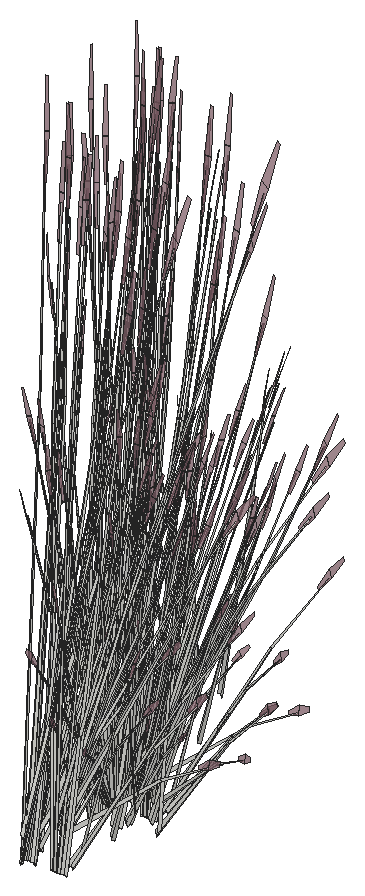
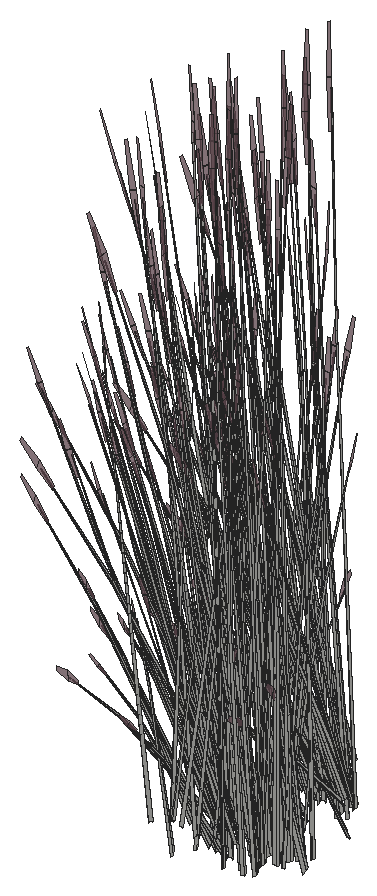
# SketchUp Ruby script. Lengths in inches.
U = 1.inch
M = Sketchup.active_model
def pt(a) = Geom::Point3d.new(a.map { |v| v * U })
def face(e, loops, mat)
  f = e.add_face(loops[0].map { |a| pt(a) })
  loops[1..].each { |l| e.add_face(l.map { |a| pt(a) }).erase! }
  f.material = f.back_material = mat if mat
  f
end
# faces: each face lists its corners as indices into pts; further lists are holes
def faces(e, pts, list, mat = nil) = list.each { |f| face(e, (f[0].is_a?(Array) ? f : [f]).map { |l| l.map { |i| pts[i] } }, mat) }
# xy, xz, yz: faces in a plane at the given z, y or x. An outline is a flat list of corners, or four numbers for a rectangle; further outlines are holes
def ring(l) = l.size == 4 ? [[l[0], l[1]], [l[2], l[1]], [l[2], l[3]], [l[0], l[3]]] : l.each_slice(2).to_a
def flat(e, list, mat, &to3) = list.each { |f| face(e, (f[0].is_a?(Array) ? f : [f]).map { |l| ring(l).map { |u, v| to3.(u, v) } }, mat) }
def xy(e, z, list, mat = nil) = flat(e, list, mat) { |x, y| [x, y, z] }
def xz(e, y, list, mat = nil) = flat(e, list, mat) { |x, z| [x, y, z] }
def yz(e, x, list, mat = nil) = flat(e, list, mat) { |y, z| [x, y, z] }
def lines(e, pts, list) = list.each { |a, b| e.add_line(pt(pts[a]), pt(pts[b])) }
# prism: a flat outline (further loops are holes) pulled along v
def prism(e, loops, v, mat = nil)
  f = face(e, loops, mat); d = Geom::Vector3d.new(v.map { |x| x * U })
  f.pushpull(f.normal.samedirection?(d) ? d.length : -d.length)
end
def box(e, o, s, mat = nil) = prism(e, [[o, [o[0] + s[0], o[1], o[2]], [o[0] + s[0], o[1] + s[1], o[2]], [o[0], o[1] + s[1], o[2]]]], [0, 0, s[2]], mat)
def at(x, y, z, deg = 0) = Geom::Transformation.translation(pt([x, y, z])) * Geom::Transformation.rotation(ORIGIN, Z_AXIS, deg.degrees)
def axes(o, x, y, z) = Geom::Transformation.new([*x, 0, *y, 0, *z, 0, *pt(o).to_a, 1])
def part(name) = M.definitions.add(name)
# library, detail: a bought-in or finely detailed component or shape, given as its bounding box
def library(name, o, s) = part(name).tap { |d| box(d.entities, o, s) }
def detail(e, o, s) = box(e.add_group.entities, o, s)
def put(e, d, t, mat = nil) = e.add_instance(d, t).tap { |i| i.material = mat if mat }
def group(e, t, mat = nil) = e.add_group.tap { |g| g.transformation = t; g.material = mat if mat }.entities
root = M.entities
M.materials.add("LightPink_Translucent").color = [144, 107, 117]
M.materials["LightPink_Translucent"].alpha = 0.75
c1 = part("blade")
p = [[2.15,0.21,22],[0,0.17,0],[0.09,0.45,0],[2.18,0.31,22],[2.29,0.31,22],[0.38,0.45,0],
  [2.48,0.24,33],[2.49,0.24,33],[2.48,0.22,33]]
faces(c1.entities,p,[[0,1,2,3],[4,5,2,3],[6,3,4,7],[8,0,3,6]])
c2 = part("seeds")
p = [[0.3,-0.1,1.38],[-0.01,-0.03,1.59],[-0.01,-0.03,0.03],[0.14,-0.07,-0.07],[0.29,-0.03,3],[0.15,0.01,3.11]]
faces(c2.entities,p,[[0,1,2,3],[1,0,4,5]],"LightPink_Translucent")
c3 = part("blade with seeds")
put(c3.entities,c1,at(0,0,0))
put(c3.entities,c2,axes([2.4,0.25,30.99],[1.5799,-0.05474,1.17369],[-0.12525,1.92788,0.29478],[-0.07173,-0.02425,1.56792]))
put(root,c3,axes([345.67,83.73,4.59],[0,0.75458,-0.05637],[-1.11865,0,0],[0,0.02371,1.79368]))
put(root,c3,axes([345.75,83.19,4.5],[0.53742,0.54764,-0.44739],[-0.81403,0.38564,0.21531],[0.17391,0.06776,1.43643]))
put(root,c3,axes([349.38,85.51,6.22],[-0.17122,-0.54847,-0.03492],[0.80929,-0.12609,-0.15832],[0.169,0.03477,0.52218]))
put(root,c3,axes([347.28,85.49,7.33],[0.0479,-0.66354,-0.1216],[0.90696,0.01814,-0.67495],[0.3493,0.04609,1.02557]))
put(root,c3,axes([348.11,83.72,4.77],[0,-0.65246,0.49651],[1.00089,0,0],[0,0.1486,1.57504]))
put(root,c3,axes([346.21,83.53,4.91],[0.83351,-0.19028,0.1448],[0.29189,0.54335,-0.41347],[0,0.11958,1.26744]))
put(root,c3,axes([347.14,85.23,7.34],[-0.50902,-0.40851,0.35414],[0.58122,-0.38671,-0.4572],[0.29531,0.05884,0.87481]))
put(root,c3,axes([349.31,84.85,4.88],[-0.21545,-0.16047,1.43002],[0.28033,-0.53085,-0.30754],[0.43591,0.07191,0.61141]))
put(root,c3,axes([345.45,85.44,4.5],[0.90188,0.29293,0],[-0.43405,0.60866,0],[0,0,1.74954]))
put(root,c3,axes([346.1,91.12,4.88],[-0.25429,0.13207,1.43002],[-0.76157,-0.23115,-0.30754],[0.14117,-0.28747,0.61141]))
put(root,c3,axes([348.07,85.1,7.01],[0.19191,-0.01103,1.74944],[0.52639,-0.5069,-0.27667],[0.34136,0.06691,0.14031]))
put(root,c3,axes([347.33,85.17,7.27],[0.89428,0.01571,-0.71045],[-0.06006,0.66153,0.08574],[0.37886,0.06981,1.00501]))
put(root,c3,axes([346.72,92.1,7.27],[0.02328,-0.60353,-0.71045],[0.98022,0.04053,0.08574],[0.10344,-0.25568,1.00501]))
put(root,c3,axes([348.09,91.16,7.01],[-0.00864,-0.12985,1.74944],[-0.72937,-0.3753,-0.27667],[0.11277,-0.2275,0.14031]))
put(root,c3,axes([345.62,91.79,6.17],[-0.16657,0.22426,1.71376],[-0.69879,-0.4641,0.13857],[0.31524,-0.28926,0.73262]))
put(root,c3,axes([347.89,90.6875,7],[-0.09085,0.04984,1.77383],[-0.89014,-0.16814,-0.16761],[-0.03222,-0.21748,0.31391]))
put(root,c3,axes([345.13,85.1875,4.58],[0.38895,0.74956,-0.06012],[-1.11135,0.26265,0],[0.01358,0.02618,1.72173]))
put(root,c3,axes([348.79,83.83,4.67],[1.11865,0,0],[0,0.72922,-0.51607],[0,0.16609,1.63711]))
put(root,c3,axes([345.16,90.07,5.06],[0.11476,0.38047,1.1486],[-0.63664,-0.21072,0.84392],[0.06851,-0.19481,0.25299]))
put(root,c3,axes([348.34,84.21,4.49],[-1.1181,-0.00522,-0.04976],[0,-0.72922,0.49943],[-0.03514,0.166,1.58352]))
put(root,c3,axes([345.92,83.57,4.96],[1.00749,0.31132,-0.29095],[-0.48511,0.65709,-0.50002],[0.03166,0.16133,1.59708]))
put(root,c3,axes([346.52,91.9,6.97],[-0.64041,-0.4384,-0.51099],[0.67652,-0.38394,-0.3958],[0.09744,-0.22274,0.97773]))
put(root,c3,axes([347.87,85.45,6.82],[0.50902,0.40851,-0.35414],[-0.58122,0.38671,0.4572],[0.29531,0.05884,0.87481]))
put(root,c3,axes([348.11,84.3125,4.32],[-0.62448,0.40708,-0.30978],[-0.62448,-0.40708,0.30978],[0,0.13112,1.38974]))
put(root,c3,axes([347.61,85.6,7.02],[-0.04505,0.49615,0.0643],[-0.68022,-0.0136,0.50621],[0.26056,0.05192,0.77189]))
put(root,c3,axes([345.81,84.06,4.5],[-0.43405,0.58792,-0.44739],[-0.90188,-0.28295,0.21531],[0,0.13553,1.43643]))
put(root,c3,axes([347.67,85.45,7.03],[-0.65964,0.42992,0.48003],[-0.5689,-0.45657,0.3958],[0.30948,0.0793,0.9933]))
put(root,c3,axes([345.12,91.24,7.03],[0.88151,0.17057,0.48003],[-0.30143,0.56078,0.3958],[-0.05297,-0.22053,0.9933]))
put(root,c3,axes([347.19,92.13,7.33],[-0.98321,-0.03233,-0.1216],[0.02687,-0.61208,-0.67495],[0.0683,-0.23574,1.02557]))
put(root,c3,axes([347.12,91.73,6.82],[0.60531,-0.34352,-0.35414],[0.573,0.39225,0.4572],[0.08718,-0.19929,0.87481]))
put(root,c3,axes([345.35,91.2,7.02],[0.6592,-0.22175,0.0643],[0.32265,0.40436,0.50621],[-0.06366,-0.17825,0.77189]))
put(root,c3,axes([345.57,85.94,7.34],[-0.13817,-0.52554,0.35414],[0.78985,-0.13877,-0.4572],[0.21215,0.1506,0.87481]))
put(root,c3,axes([348.54,84.33,4.3125],[0,0.65246,-0.49651],[-1.00089,0,0],[0,0.1486,1.57504]))
put(root,c3,axes([346.04,84.4,6.17],[-0.3323,-0.11241,1.71376],[0.68769,-0.4716,0.13857],[0.42861,0.21275,0.73262]))
put(root,c3,axes([346.1,82.92,6.77],[-0.77304,-0.33901,1.38283],[0.81626,-0.52782,0.59665],[0.24941,0.31809,1.33663]))
put(root,c3,axes([347.27,85.68,5.06],[-0.5037,-0.18761,1.1486],[0.6504,-0.19062,0.84392],[0.17543,0.16147,0.25299]))
put(root,c3,axes([345.5,86.22,7.33],[0.53309,-0.55848,-0.1216],[0.77201,0.32175,-0.67495],[0.26836,0.15779,1.02557]))
put(root,c3,axes([347.88,91.53,3.79],[-0.1339,-0.0514,1.76342],[-0.34394,-0.57425,-0.26939],[0.23202,-0.15583,0.30037]))
put(root,c3,axes([344.8,86.68,7],[0.00265,-0.07899,1.77383],[0.76665,-0.34851,-0.16761],[0.2663,0.12439,0.31391]))
put(root,c3,axes([347.41,86.375,3.79],[0.06518,-0.0942,1.76342],[0.82057,-0.27742,-0.26939],[0.24877,0.14358,0.30037]))
put(root,c3,axes([346.33,84.24,4.39],[0.32803,0.59738,-0.69212],[-0.94492,0.21515,-0.18165],[0.03626,0.20229,1.52773]))
put(root,c3,axes([347.12,91.87,7.03],[0.63704,0.44518,0.48003],[-0.67652,0.38394,0.3958],[0.11751,-0.20886,0.9933]))
put(root,c3,axes([347.36,91.91,7.02],[0.73517,0.0304,0.0643],[-0.02016,0.45906,0.50621],[0.07693,-0.17585,0.77189]))
put(root,c3,axes([346.13,85.9375,6.97],[0.88277,-0.1551,-0.51099],[0.15442,0.58737,-0.3958],[0.23711,0.16832,0.97773]))
put(root,c3,axes([343.68,86.03,7.34],[0.2697,-0.50175,0.35414],[0.78684,0.14635,-0.4572],[0.07215,0.20201,0.87481]))
put(root,c3,axes([346.81,92.22,7.34],[-0.60531,0.34352,0.35414],[-0.573,-0.39225,-0.4572],[0.08718,-0.19929,0.87481]))
put(root,c3,axes([347.875,93.15,7.27],[0.4673,-0.51481,-0.71045],[0.81887,0.36587,0.08574],[0.27902,-0.18652,1.00501]))
put(root,c3,axes([342.82,91.65,4.67],[-0.55932,-0.6538,0],[0.93577,-0.36461,-0.51607],[0.21313,-0.08304,1.63711]))
put(root,c3,axes([347.85,92.91,6.97],[-0.22982,-0.59576,-0.51099],[0.87033,-0.10422,-0.3958],[0.24941,-0.16002,0.97773]))
put(root,c3,axes([347.35,86.53,4.96],[-0.57368,-0.02046,1.0506],[0.37886,-0.43461,0.58006],[0.22663,0.15441,0.8241]))
put(root,c3,axes([345.7,86.42,7.02],[-0.4066,0.41448,0.0643],[-0.57901,-0.24131,0.50621],[0.18719,0.13288,0.77189]))
put(root,c3,axes([348.26,93.33,7.33],[-0.82753,-0.35977,-0.1216],[0.47675,-0.52101,-0.67495],[0.2338,-0.18111,1.02557]))
put(root,c3,axes([344.74,87.82,7.9375],[0.61821,-0.37431,-0.06488],[0.56645,0.40995,-0.29416],[0.03988,0.11616,0.97024]))
put(root,c3,axes([345.87,86.3,7.03],[-0.88979,0.14973,0.48003],[-0.15442,-0.58737,0.3958],[0.20926,0.17311,0.9933]))
put(root,c3,axes([345.48,85.48,4.88],[0.01579,-0.21629,1.43002],[0.75442,-0.24159,-0.30754],[0.23289,0.25887,0.61141]))
put(root,c3,axes([343.58,91.55,4.3125],[0.83726,-0.32623,-0.49651],[0.50045,0.58498,0],[0.19069,-0.0743,1.57504]))
put(root,c3,axes([348.55,92.67,4.88],[-0.31959,-0.01933,1.43002],[-0.32741,-0.51843,-0.30754],[0.39262,-0.14666,0.61141]))
put(root,c3,axes([350.3,93.18,7],[-0.11685,-0.00496,1.77383],[-0.48522,-0.53096,-0.16761],[0.19486,-0.17458,0.31391]))
put(root,c3,axes([343.42,86.24,7.33],[0.87543,-0.30377,-0.1216],[0.4302,0.53915,-0.67495],[0.1155,0.2272,1.02557]))
put(root,c3,axes([344.57,92.88,4.35],[0.60257,-0.49041,-0.62353],[0.74854,0.44469,-0.16365],[0.24146,-0.12234,1.37633]))
put(root,c3,axes([348.92,91.72,5.06],[-0.29798,0.33213,1.1486],[-0.25612,-0.44624,0.84392],[0.24611,-0.11182,0.25299]))
put(root,c3,axes([343.58,86.36,3.79],[0.14478,-0.0355,1.76342],[0.8709,0.19542,-0.26939],[0.02547,0.22025,0.30037]))
put(root,c3,axes([348.49,92.97,6.82],[0.77872,-0.09325,-0.35414],[0.20563,0.53305,0.4572],[0.22316,-0.14318,0.87481]))
put(root,c3,axes([343.53,93.74,4.5],[0.43405,-0.58792,-0.44739],[0.90188,0.28295,0.21531],[0,-0.13553,1.43643]))
put(root,c3,axes([343.92,93.45,4.96],[-0.10425,-0.7445,-0.29095],[1.08575,-0.04502,-0.50002],[0.19119,-0.09917,1.59708]))
put(root,c3,axes([344.17,86.21,6.97],[0.87941,0.16356,-0.51099],[-0.30143,0.56078,-0.3958],[0.08064,0.22578,0.97773]))
put(root,c3,axes([344.67,85.05,6.17],[-0.2045,-0.20949,1.71376],[0.94495,-0.17636,0.13857],[0.21357,0.32887,0.73262]))
put(root,c3,axes([347.86,93.28,7.34],[-0.77872,0.09325,0.35414],[-0.20563,-0.53305,-0.4572],[0.22316,-0.14318,0.87481]))
put(root,c3,axes([343.77,86.55,6.82],[-0.2697,0.50175,-0.35414],[-0.78684,-0.14635,0.4572],[0.07215,0.20201,0.87481]))
put(root,c3,axes([343.78,91.8,4.32],[0.83462,0.16144,-0.30978],[-0.21015,0.56852,0.30978],[0.16826,-0.06556,1.38974]))
put(root,c3,axes([348.5625,93.2,7.02],[0.61415,0.2744,0.0643],[-0.35756,0.39076,0.50621],[0.1969,-0.12633,0.77189]))
put(root,c3,axes([348.39,93.08,7.03],[0.22187,0.60049,0.48003],[-0.87033,0.10422,0.3958],[0.25651,-0.14123,0.9933]))
put(root,c3,axes([350.74,93.8125,7.01],[0.12414,-0.09938,1.74944],[-0.15889,-0.60963,-0.27667],[0.31148,-0.11559,0.14031]))
put(root,c3,axes([343.85,86.1,7.27],[0.42698,0.53052,-0.71045],[-0.87893,0.29566,0.08574],[0.09984,0.25633,1.00501]))
put(root,c3,axes([343.21,87.44,7.01],[0.1134,0.10507,1.74944],[0.91515,0.04128,-0.27667],[0.09203,0.23172,0.14031]))
put(root,c3,axes([344.0625,94.04,4.73],[1.00799,0.31623,0.24065],[-0.48511,0.65709,0.50002],[0,-0.15147,1.60543]))
put(root,c3,axes([343.74,93.6,5.01],[-0.97146,0.04028,0.44739],[-0.08785,-0.66859,-0.21531],[0.17391,-0.06776,1.43643]))
put(root,c3,axes([348.29,94.74,7.33],[-0.45012,-0.59081,-0.1216],[0.79888,-0.29033,-0.67495],[0.33665,-0.07795,1.02557]))
put(root,c3,axes([348.26,94.23,6.97],[0.24236,-0.59349,-0.51099],[0.83094,0.20343,-0.3958],[0.33455,-0.05442,0.97773]))
put(root,c3,axes([346.94,91.8125,4.67],[0.55932,-0.6538,0],[0.93577,0.36461,-0.51607],[0.21313,0.08304,1.63711]))
put(root,c3,axes([349.14,94.4,4.28],[-0.57619,0.0783,1.41583],[-0.09171,-0.62326,0.08104],[0.40356,-0.09434,0.80566]))
put(root,c3,axes([350.19,93.84,4.55],[-0.55463,-0.41721,-0.06488],[0.60744,-0.38228,-0.29416],[0.17212,-0.02691,0.97024]))
put(root,c3,axes([345.1,93.9,4.5],[0,-0.75495,0],[1.11865,0,0],[0,0,1.79456]))
put(root,c3,axes([346.46,92.15,4.77],[-0.83726,-0.32623,0.49651],[0.50045,-0.58498,0],[0.19069,0.0743,1.57504]))
put(root,c3,axes([348.1,94.45,7.27],[0.78611,-0.28816,-0.71045],[0.4381,0.59317,0.08574],[0.37982,-0.06738,1.00501]))
put(root,c3,axes([344.57,93.42,4.65],[-0.74176,0.59212,0.45755],[-0.88124,-0.52269,0.17955],[0.17882,-0.05909,1.58856]))
put(root,c3,axes([343.29,92.45,4.77],[-0.25843,0.64844,0.17642],[-0.9457,-0.1835,0.35086],[0.16336,-0.00316,1.60407]))
put(root,c3,axes([347.98,94.56,7.34],[-0.74348,-0.18202,0.35414],[0.21685,-0.53102,-0.4572],[0.29933,-0.04869,0.87481]))
put(root,c3,axes([342.89,92.97,3.89],[-0.88056,0.26122,1.28929],[-0.28027,-0.74951,0.50096],[0.54072,0.01247,1.46642]))
put(root,c3,axes([345.26,93.17,4.91],[0.17258,-0.58229,0.1448],[0.84319,0.10108,-0.41347],[0.15345,0.05979,1.26744]))
put(root,c3,axes([349.77,93.99,3.79],[-0.04675,-0.09906,1.76342],[0.32428,-0.57943,-0.26939],[0.32711,-0.00833,0.30037]))
put(root,c3,axes([344.9,93.32,5.01],[-0.53742,-0.54764,0.44739],[0.81403,-0.38564,-0.21531],[0.17391,0.06776,1.43643]))
put(root,c3,axes([345.17,93.36,4.96],[0.90324,-0.43318,-0.29095],[0.60064,0.61207,-0.50002],[0.22285,0.06216,1.59708]))
put(root,c3,axes([348.76,94.5,6.82],[0.74348,0.18202,-0.35414],[-0.21685,0.53102,0.4572],[0.29933,-0.04869,0.87481]))
put(root,c3,axes([347.45,92.21,4.3125],[0.83726,0.32623,-0.49651],[-0.50045,0.58498,0],[0.19069,0.0743,1.57504]))
put(root,c3,axes([345.86,94.07,4.5],[1.00089,0,0],[0,0.67548,0],[0,0,1.78407]))
put(root,c3,axes([346.15,92.48,4.77],[-0.96132,0.17317,0.17642],[-0.23737,-0.64447,0.35086],[0.08574,0.0939,1.60407]))
put(root,c3,axes([346.74,93.84,6.17],[-0.37107,0.01478,1.71376],[0.24616,-0.64047,0.13857],[0.5288,0.03961,0.73262]))
put(root,c3,axes([347.22,92.45,4.32],[0.21015,0.56852,-0.30978],[-0.83462,0.16144,0.30978],[0.16826,0.06556,1.38974]))
put(root,c3,axes([348.66,94.72,7.02],[0.32857,0.44488,0.0643],[-0.59916,0.21775,0.50621],[0.26412,-0.04296,0.77189]))
put(root,c3,axes([345.54,93.72,4.67],[-1.13071,-0.13747,0.49198],[0.23011,-0.77639,0.19306],[0.16524,0.07497,1.70813]))
put(root,c3,axes([348.59,94.57,7.03],[-0.25275,0.59491,0.48003],[-0.83094,-0.20343,0.3958],[0.32677,-0.03575,0.9933]))
put(root,c3,axes([344.64,95.64,4.5],[-0.29189,-0.56252,0],[0.83351,-0.19699,0],[0,0,1.54371]))
put(root,c3,axes([345.73,95.5625,4.48],[0.93921,-0.22138,-0.19198],[0.33003,0.6377,0.00008],[0.10367,-0.02447,1.73897]))
put(root,c3,axes([345.84,94.36,4.51],[0.62448,0.42144,0],[-0.62448,0.42144,0],[0,0,1.69266]))
put(root,c3,axes([347.53,94.17,4.77],[-0.70288,-0.47526,0.17642],[0.70832,-0.46097,0.35086],[-0.07763,0.09706,1.60407]))
put(root,c3,axes([346.23,93.46,4.35],[0.9306,0.10697,-0.62353],[-0.19638,0.65984,-0.16365],[0.27771,0.07995,1.37633]))
put(root,c3,axes([350.34,94.61,5.06],[-0.55274,0.10771,1.1486],[0.26018,-0.44517,0.84392],[0.29323,0.03046,0.25299]))
put(root,c3,axes([345.83,93.86,5.01],[0.43405,-0.58792,0.44739],[0.90188,0.28295,-0.21531],[0,0.13553,1.43643]))
put(root,c3,axes([350.09,96.49,7],[-0.08089,-0.05712,1.77383],[0.17695,-0.61228,-0.16761],[0.31864,-0.03912,0.31391]))
put(root,c3,axes([345.67,94.2,4.59],[0,0.75458,-0.05637],[-1.11865,0,0],[0,0.02371,1.79368]))
put(root,c3,axes([345.75,93.67,4.5],[0.53742,0.54764,-0.44739],[-0.81403,0.38564,0.21531],[0.17391,0.06776,1.43643]))
put(root,c3,axes([349.38,95.98,6.22],[-0.17122,-0.54847,-0.03492],[0.80929,-0.12609,-0.15832],[0.169,0.03477,0.52218]))
put(root,c3,axes([347.28,95.96,7.33],[0.0479,-0.66354,-0.1216],[0.90696,0.01814,-0.67495],[0.3493,0.04609,1.02557]))
put(root,c3,axes([348.11,94.19,4.77],[0,-0.65246,0.49651],[1.00089,0,0],[0,0.1486,1.57504]))
put(root,c3,axes([346.21,94,4.91],[0.83351,-0.19028,0.1448],[0.29189,0.54335,-0.41347],[0,0.11958,1.26744]))
put(root,c3,axes([347.14,95.7,7.34],[-0.50902,-0.40851,0.35414],[0.58122,-0.38671,-0.4572],[0.29531,0.05884,0.87481]))
put(root,c3,axes([346.1,101.1875,8.59],[-0.25429,0.13207,1.43002],[-0.76157,-0.23115,-0.30754],[0.14117,-0.28747,0.61141]))
put(root,c3,axes([349.31,95.32,4.88],[-0.21545,-0.16047,1.43002],[0.28033,-0.53085,-0.30754],[0.43591,0.07191,0.61141]))
put(root,c3,axes([345.45,95.91,4.5],[0.90188,0.29293,0],[-0.43405,0.60866,0],[0,0,1.74954]))
put(root,c3,axes([348.07,95.57,7.01],[0.19191,-0.01103,1.74944],[0.52639,-0.5069,-0.27667],[0.34136,0.06691,0.14031]))
put(root,c3,axes([346.72,102.17,10.98],[0.02328,-0.60353,-0.71045],[0.98022,0.04053,0.08574],[0.10344,-0.25568,1.00501]))
put(root,c3,axes([345.62,101.86,9.875],[-0.16657,0.22426,1.71376],[-0.69879,-0.4641,0.13857],[0.31524,-0.28926,0.73262]))
put(root,c3,axes([347.33,95.65,7.27],[0.89428,0.01571,-0.71045],[-0.06006,0.66153,0.08574],[0.37886,0.06981,1.00501]))
put(root,c3,axes([345.16,100.14,8.77],[0.11476,0.38047,1.1486],[-0.63664,-0.21072,0.84392],[0.06851,-0.19481,0.25299]))
put(root,c3,axes([346.52,101.97,10.68],[-0.64041,-0.4384,-0.51099],[0.67652,-0.38394,-0.3958],[0.09744,-0.22274,0.97773]))
put(root,c3,axes([345.13,95.66,4.58],[0.38895,0.74956,-0.06012],[-1.11135,0.26265,0],[0.01358,0.02618,1.72173]))
put(root,c3,axes([348.79,94.3,4.67],[1.11865,0,0],[0,0.72922,-0.51607],[0,0.16609,1.63711]))
put(root,c3,axes([348.34,94.68,4.49],[-1.1181,-0.00522,-0.04976],[0,-0.72922,0.49943],[-0.03514,0.166,1.58352]))
put(root,c3,axes([345.92,94.04,4.96],[1.00749,0.31132,-0.29095],[-0.48511,0.65709,-0.50002],[0.03166,0.16133,1.59708]))
put(root,c3,axes([347.87,95.92,6.82],[0.50902,0.40851,-0.35414],[-0.58122,0.38671,0.4572],[0.29531,0.05884,0.87481]))
put(root,c3,axes([348.11,94.78,4.32],[-0.62448,0.40708,-0.30978],[-0.62448,-0.40708,0.30978],[0,0.13112,1.38974]))
put(root,c3,axes([347.61,96.07,7.02],[-0.04505,0.49615,0.0643],[-0.68022,-0.0136,0.50621],[0.26056,0.05192,0.77189]))
put(root,c3,axes([345.81,94.53,4.5],[-0.43405,0.58792,-0.44739],[-0.90188,-0.28295,0.21531],[0,0.13553,1.43643]))
put(root,c3,axes([347.12,101.8,10.53],[0.60531,-0.34352,-0.35414],[0.573,0.39225,0.4572],[0.08718,-0.19929,0.87481]))
put(root,c3,axes([347.67,95.92,7.03],[-0.65964,0.42992,0.48003],[-0.5689,-0.45657,0.3958],[0.30948,0.0793,0.9933]))
put(root,c3,axes([345.57,96.41,7.34],[-0.13817,-0.52554,0.35414],[0.78985,-0.13877,-0.4572],[0.21215,0.1506,0.87481]))
put(root,c3,axes([348.54,94.8,4.3125],[0,0.65246,-0.49651],[-1.00089,0,0],[0,0.1486,1.57504]))
put(root,c3,axes([346.04,94.87,6.17],[-0.3323,-0.11241,1.71376],[0.68769,-0.4716,0.13857],[0.42861,0.21275,0.73262]))
put(root,c3,axes([346.1,93.39,6.77],[-0.77304,-0.33901,1.38283],[0.81626,-0.52782,0.59665],[0.24941,0.31809,1.33663]))
put(root,c3,axes([347.88,101.6,7.49],[-0.1339,-0.0514,1.76342],[-0.34394,-0.57425,-0.26939],[0.23202,-0.15583,0.30037]))
put(root,c3,axes([347.27,96.15,5.06],[-0.5037,-0.18761,1.1486],[0.6504,-0.19062,0.84392],[0.17543,0.16147,0.25299]))
put(root,c3,axes([345.5,96.6875,7.33],[0.53309,-0.55848,-0.1216],[0.77201,0.32175,-0.67495],[0.26836,0.15779,1.02557]))
put(root,c3,axes([347.875,103.21,10.98],[0.4673,-0.51481,-0.71045],[0.81887,0.36587,0.08574],[0.27902,-0.18652,1.00501]))
put(root,c3,axes([342.82,101.72,8.375],[-0.55932,-0.6538,0],[0.93577,-0.36461,-0.51607],[0.21313,-0.08304,1.63711]))
